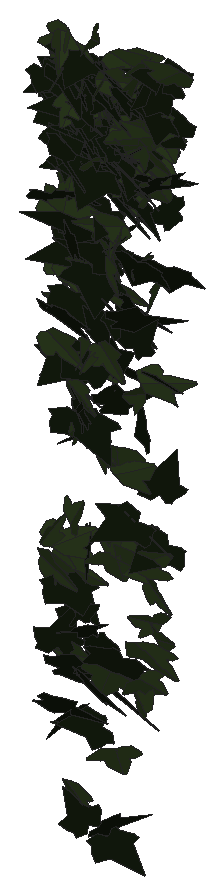
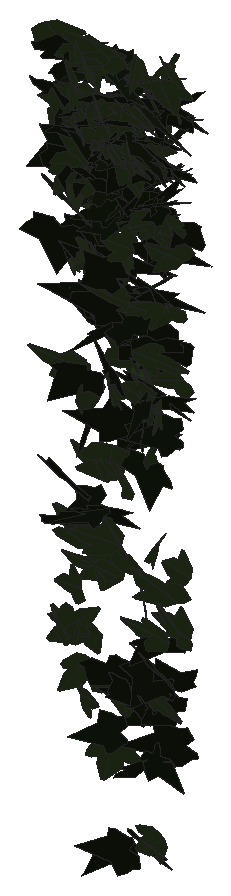
# SketchUp Ruby script. Lengths in millimetres.
U = 1.mm
M = Sketchup.active_model
def pt(a) = Geom::Point3d.new(a.map { |v| v * U })
def face(e, loops, mat)
  f = e.add_face(loops[0].map { |a| pt(a) })
  loops[1..].each { |l| e.add_face(l.map { |a| pt(a) }).erase! }
  f.material = f.back_material = mat if mat
  f
end
# faces: each face lists its corners as indices into pts; further lists are holes
def faces(e, pts, list, mat = nil) = list.each { |f| face(e, (f[0].is_a?(Array) ? f : [f]).map { |l| l.map { |i| pts[i] } }, mat) }
# xy, xz, yz: faces in a plane at the given z, y or x. An outline is a flat list of corners, or four numbers for a rectangle; further outlines are holes
def ring(l) = l.size == 4 ? [[l[0], l[1]], [l[2], l[1]], [l[2], l[3]], [l[0], l[3]]] : l.each_slice(2).to_a
def flat(e, list, mat, &to3) = list.each { |f| face(e, (f[0].is_a?(Array) ? f : [f]).map { |l| ring(l).map { |u, v| to3.(u, v) } }, mat) }
def xy(e, z, list, mat = nil) = flat(e, list, mat) { |x, y| [x, y, z] }
def xz(e, y, list, mat = nil) = flat(e, list, mat) { |x, z| [x, y, z] }
def yz(e, x, list, mat = nil) = flat(e, list, mat) { |y, z| [x, y, z] }
def lines(e, pts, list) = list.each { |a, b| e.add_line(pt(pts[a]), pt(pts[b])) }
# prism: a flat outline (further loops are holes) pulled along v
def prism(e, loops, v, mat = nil)
  f = face(e, loops, mat); d = Geom::Vector3d.new(v.map { |x| x * U })
  f.pushpull(f.normal.samedirection?(d) ? d.length : -d.length)
end
def box(e, o, s, mat = nil) = prism(e, [[o, [o[0] + s[0], o[1], o[2]], [o[0] + s[0], o[1] + s[1], o[2]], [o[0], o[1] + s[1], o[2]]]], [0, 0, s[2]], mat)
def at(x, y, z, deg = 0) = Geom::Transformation.translation(pt([x, y, z])) * Geom::Transformation.rotation(ORIGIN, Z_AXIS, deg.degrees)
def axes(o, x, y, z) = Geom::Transformation.new([*x, 0, *y, 0, *z, 0, *pt(o).to_a, 1])
def part(name) = M.definitions.add(name)
# library, detail: a bought-in or finely detailed component or shape, given as its bounding box
def library(name, o, s) = part(name).tap { |d| box(d.entities, o, s) }
def detail(e, o, s) = box(e.add_group.entities, o, s)
def put(e, d, t, mat = nil) = e.add_instance(d, t).tap { |i| i.material = mat if mat }
def group(e, t, mat = nil) = e.add_group.tap { |g| g.transformation = t; g.material = mat if mat }.entities
root = M.entities
M.materials.add("efeu1").color = [18, 25, 13]
M.materials.add("efeu2").color = [43, 57, 29]
c1 = part("ivyleaf_9")
p = [[39.1,54.8,31.7],[34.5,51.8,30.2],[-5.3,25.2,17.3],[-17.9,28.3,20.9],[-21.6,21.7,17],[-20.2,4.3,5.3],
  [-22.9,-0.3,2.5],[-17.1,-4,-0.6],[-2,-2.1,-1.2],[-0.7,-15.4,-10.1],[16.6,-22.3,-16.7],[21.1,-15.1,-12.5],
  [32.7,-10.7,-11],[46.1,-1.8,-6.6],[30.8,11.2,3.8]]
faces(c1.entities,p,[[0,1,2,3,4,5,6,7,8,9,10,11,12,13,14]],"efeu1")
c2 = part("ivyleaf_10")
p = [[0,12.8,-0.8],[-1.5,51.3,-10.9],[-4.9,51,-11.6],[-13.6,26.5,-7.3],[-13.2,15.9,-4.6],[-21.1,19.3,-7.2],
  [-29.5,16.3,-8.3],[-29.2,8.3,-6.2],[-19.7,-9.8,0.5],[-7.6,-13,4],[1,-12.2,5.8],[-0.4,51.1,-11.1],
  [-1.5,51.1,-10.9],[1,-12.4,5.9],[16.9,-12.4,3.5],[35.1,9.1,-5.1],[35,12.9,-6.1],[20.5,16.4,-4.9],
  [15.8,15,-3.8],[15.3,27.6,-7.1],[12.8,31.3,-7.8]]
faces(c2.entities,p,[[0,1,2,3,4,5,6,7,8,9,10],[11,12,0,13,14,15,16,17,18,19,20]],"efeu2")
put(root,c1,axes([2883.6,930,998.6],[-0.63134,-0.54805,-0.68858],[0.6758,0.58996,-0.64063],[1.53254,-0.48593,-0.00117]))
put(root,c1,axes([2814.2,927.9,1572.8],[0.42364,-0.6267,-0.48664],[-0.1479,0.48577,-0.66114],[1.50284,0.22447,0.07211]))
put(root,c1,axes([2824.3,923.5,489.8],[1.26667,0.04328,0.44833],[0.8493,0.04515,-0.66682],[-0.11628,0.80119,0.01336]))
put(root,c1,axes([2901.8,943.8,1419.4],[-1.00985,-0.67232,0.03547],[-0.0298,-0.03283,-0.85644],[1.281,-0.53078,0.00804]))
put(root,c2,axes([2826.4,921.6,772.8],[0.15116,-0.68397,0.61887],[-0.19573,0.61072,0.68816],[-1.74456,-0.12778,-0.02359]))
put(root,c1,axes([2953.8,925.9,1588.4],[1.11488,-0.41864,-0.46192],[-0.58225,0.35923,-0.71354],[1.03377,0.65382,0.09628]))
put(root,c2,axes([2840.4,927.7,1579.9],[0.4073,-0.77882,-0.38187],[-0.19853,0.36736,-0.80768],[1.63886,0.23806,-0.00294]))
put(root,c2,axes([2863.9,938.3,1531.9],[0.85208,0.61092,-0.37702],[-0.39134,-0.31658,-0.75716],[-1.30903,0.4923,-0.01905]))
put(root,c1,axes([2870.3,948.8,1520.5],[-0.85456,-0.2473,0.7023],[-1.02719,-0.45686,-0.50594],[0.97619,-0.69722,0.08242]))
put(root,c1,axes([2880.7,944,534.4],[0.58926,-0.49402,0.63243],[0.67074,-0.5253,-0.58287],[1.37218,0.46892,0.01333]))
put(root,c2,axes([2951.3,930.1,444.2],[-1.09314,-0.67103,-0.23331],[0.27125,0.18508,-0.88321],[1.32462,-0.59167,-0.01168]))
put(root,c1,axes([2871.9,924.2,1284.3],[0.04835,-0.26099,0.79603],[-0.14077,0.79259,0.26222],[-1.58814,-0.0782,0.00099]))
put(root,c2,axes([2990.5,933.8,779],[-1.40972,-0.27616,0.56116],[0.99911,0.19828,0.79051],[-0.64702,0.90787,-0.00196]))
put(root,c2,axes([2863.7,950.9,969.6],[-0.2876,0.2348,0.91607],[0.70199,-0.83959,0.27604],[1.65728,0.39638,0.04205]))
put(root,c2,axes([2860.2,943.9,1033.5],[-0.49701,0.25279,-0.71399],[0.86298,-0.55277,-0.36156],[-1.15467,-0.52194,0.03711]))
put(root,c1,axes([2974.1,948.1,840.1],[-1.35807,-0.37116,0.27644],[-0.45189,-0.14246,-0.80417],[0.75603,-0.75187,0.01591]))
put(root,c2,axes([2939.8,945.2,1332.4],[0.87647,-0.62325,0.36788],[0.40894,-0.29863,-0.77492],[1.31528,0.50817,-0.00421]))
put(root,c1,axes([2874.6,952.1,991.3],[0.04901,0.05203,0.86048],[-0.52356,-0.81536,0.05753],[1.55488,-0.27619,-0.00775]))
put(root,c2,axes([2916.1,948.1,1260.8],[-0.47084,0.36892,-0.73202],[0.59454,-0.6645,-0.44047],[-1.44239,-0.39433,0.0574]))
put(root,c2,axes([2990.2,943.2,1512.8],[-0.86521,-0.26856,0.6914],[-1.12787,-0.35615,-0.528],[0.84892,-0.7469,0.00316]))
put(root,c2,axes([2921.7,944.8,791.3],[0.75953,-0.51959,-0.47396],[0.58047,-0.36317,0.65495],[-1.20608,-0.502,0.01675]))
put(root,c1,axes([2896.5,927.4,303.6],[-1.21674,0.2044,-0.45949],[-0.82972,0.14522,0.67118],[0.47713,0.7738,-0.00459]))
put(root,c2,axes([2834.7,943.6,1628.3],[0.2442,0.75026,-0.38641],[-0.09263,-0.38362,-0.761],[-1.60347,0.13642,-0.01488]))
put(root,c1,axes([2873.3,931.5,1021.3],[1.00187,-0.39496,-0.54441],[-0.74918,0.37964,-0.65605],[1.03793,0.65526,0.05195]))
put(root,c2,axes([2849.6,935.9,1348.8],[1.69845,-0.0937,-0.04669],[0.08838,-0.00485,0.89732],[-0.17857,-0.89363,0.00002]))
put(root,c2,axes([2820.2,940.1,1106.6],[0.93583,-0.02456,0.68501],[1.30429,0.03446,-0.49069],[-0.02606,0.84252,0.04004]))
put(root,c1,axes([2829.5,932.6,1163.8],[1.59709,-0.04245,-0.15527],[-0.2952,0.00708,-0.84024],[0.08189,0.85338,-0.00075]))
put(root,c1,axes([2837.4,948.5,1442.3],[0.28172,-0.85599,0.04688],[0.01043,-0.04663,-0.86869],[1.63152,0.14811,-0.00254]))
put(root,c2,axes([2921.2,932.1,1593.4],[0.25219,-0.7053,-0.48967],[-0.0902,0.4887,-0.71674],[1.63163,0.13603,0.03606]))
put(root,c1,axes([2832.4,952.3,1561.9],[0.14112,-0.85093,0.24891],[0.16741,-0.24149,-0.85175],[1.67902,0.0956,0.06401]))
put(root,c2,axes([2867.8,946.3,1566],[0.84455,-0.69965,0.2326],[0.24622,-0.19337,-0.82849],[1.38145,0.4622,0.00547]))
put(root,c1,axes([2873.8,945.7,1317.7],[-0.68279,0.03215,-0.71065],[-0.88916,-0.61085,0.20822],[-1.02098,0.51048,0.29391]))
put(root,c1,axes([2987.2,935.7,1296.8],[1.16636,0.18657,-0.5871],[-1.06264,-0.18167,-0.64056],[-0.49536,0.82901,-0.00825]))
put(root,c2,axes([2910.5,946.9,1114.5],[0.97749,-0.20518,0.64934],[1.20621,-0.15352,-0.5498],[0.47415,0.81355,0.06002]))
put(root,c1,axes([2835.8,933.7,586.3],[-0.72,-0.35315,0.72211],[1.18478,0.3762,0.51011],[-0.96788,0.72321,0.08726]))
put(root,c1,axes([2934.8,935,287.1],[0.07191,-0.50189,-0.72315],[-0.11347,0.72069,-0.5033],[1.67144,0.07052,-0.00306]))
put(root,c2,axes([2931.1,940.1,564.4],[-1.62972,-0.1523,0.23958],[-0.44917,-0.04125,-0.86974],[0.3003,-0.88823,-0.00069]))
put(root,c2,axes([2937.6,944,1339.1],[0.55558,0.05176,-0.75248],[-1.43364,-0.02097,-0.29367],[-0.0729,0.80684,0.04064]))
put(root,c2,axes([2998,940.7,633.1],[-1.4185,0.07894,-0.51976],[0.97901,-0.07659,-0.74928],[-0.20649,-0.90542,0.01806]))
put(root,c1,axes([3025.2,955.6,815.4],[-1.22428,-0.5386,0.2061],[-0.30552,-0.12932,-0.83897],[1.05417,-0.66299,-0.00379]))
put(root,c1,axes([2841.3,937.3,547.7],[0.72496,-0.06687,0.7994],[1.5253,-0.00645,-0.38243],[0.06586,0.88549,0.05758]))
put(root,c1,axes([2828.2,931.8,1361.5],[1.45414,0.57437,-0.04188],[-0.06398,-0.02498,-0.95586],[-1.09417,0.76479,0.00023]))
put(root,c1,axes([2896.9,949.8,1238.1],[-1.19147,-0.38377,-0.42316],[0.66649,0.23817,-0.7341],[0.85899,-0.71712,-0.01735]))
put(root,c2,axes([3010.9,954.2,1259.6],[0.45099,-0.69809,0.4273],[0.31718,-0.39438,-0.73672],[1.52511,0.28845,0.02686]))
put(root,c1,axes([2957.9,932.5,1188.6],[0.73605,0.04129,0.82396],[1.48165,0.28292,-0.37958],[-0.51966,0.86513,0.08481]))
put(root,c1,axes([2848.9,950.2,1565.3],[-1.56216,0.04865,0.0752],[-0.14685,-0.03199,-0.82144],[-0.08656,-0.82362,0.03634]))
put(root,c1,axes([2977.7,940.3,1148.3],[-0.7019,0.59982,0.41627],[0.33559,-0.37938,0.70289],[1.34841,0.40664,0.04175]))
put(root,c1,axes([3002.3,961.5,1550.6],[-0.38626,-0.72127,0.44661],[0.19272,-0.47653,-0.72356],[1.60302,-0.1165,0.1946]))
put(root,c1,axes([2854.9,948.7,473.2],[-0.44054,0.56882,-0.55447],[0.41481,-0.50989,-0.61407],[-1.45378,-0.31785,-0.00719]))
put(root,c1,axes([2915.3,947,1599.6],[1.08297,-0.60883,-0.02337],[-0.01196,0.0261,-0.83324],[1.15952,0.56891,0.01323]))
put(root,c1,axes([2844.5,959,1071.5],[-1.07585,-0.54835,0.28499],[-0.3728,-0.20733,-0.78746],[1.1155,-0.59815,0.01169]))
put(root,c1,axes([2895.7,953.3,1555.3],[0.73341,-0.74928,0.17655],[0.17153,-0.15217,-0.84251],[1.45502,0.39562,0.01033]))
put(root,c1,axes([2942.1,949.2,593.5],[0.25796,0.30212,-0.80226],[-0.85908,-0.66536,-0.32683],[-1.38704,0.46829,0.05322]))
put(root,c1,axes([2965.3,944.1,850.6],[1.50653,-0.47803,-0.10684],[-0.16997,0.05879,-0.92471],[0.91661,0.79659,0.00413]))
put(root,c1,axes([2840.7,946.2,1552.8],[-0.68925,-0.3754,-0.68405],[0.89355,0.49752,-0.5216],[1.18615,-0.59293,-0.00456]))
put(root,c2,axes([2877,945,1107],[0.57076,-0.88965,-0.21557],[-0.12619,0.20514,-0.93883],[1.7376,0.30713,0.00263]))
put(root,c1,axes([2832.2,960.7,1442.8],[-0.31671,-0.83006,0.24522],[-0.08584,-0.24106,-0.84657],[1.64503,-0.17239,0.00304]))
put(root,c1,axes([2896.7,950.5,1086],[-1.69564,0.21213,0.14268],[-0.26476,0.03176,-0.91585],[-0.40822,-0.90174,0.00131]))
put(root,c2,axes([2939.6,944.5,769.8],[-1.2672,-0.61868,-0.19706],[0.27694,0.13289,-0.90889],[1.20432,-0.68154,0.00166]))
put(root,c1,axes([2856.5,962.5,1599.9],[-0.82221,-0.68704,0.20937],[0.02086,-0.25061,-0.79974],[1.36679,-0.40948,0.13815]))
put(root,c2,axes([2886.2,936.5,1082.6],[0.72199,-0.47502,0.61192],[-0.39414,0.59437,0.58977],[-1.42066,-0.4063,0.14736]))
put(root,c2,axes([2984.8,940.9,1494.5],[0.988,-0.39042,-0.56565],[-0.56333,0.51277,-0.62557],[1.18057,0.57142,0.17488]))
put(root,c2,axes([2890,957.6,1427],[0.09567,-0.79253,0.32776],[0.03504,-0.32725,-0.79412],[1.63187,0.05349,-0.00216]))
put(root,c1,axes([2932.9,950.6,1273.2],[-0.68948,0.10427,0.71846],[-1.31482,0.19728,-0.37698],[-0.42467,-0.78007,0.00069]))
put(root,c2,axes([2792,959.2,701.9],[0.01821,-0.11853,0.97857],[1.75075,-0.35055,-0.05146],[0.67408,0.91368,0.10721]))
put(root,c2,axes([2947.2,952.6,914.7],[1.11623,-0.21706,-0.6099],[1.10427,-0.18878,0.62514],[-0.54648,-0.82482,0.01743]))
put(root,c1,axes([3015.9,955.1,1590.7],[-1.453,0.21406,-0.26205],[0.49285,-0.04664,-0.79254],[-0.41451,-0.80582,-0.02374]))
put(root,c2,axes([2849.8,953.6,336.5],[-1.0113,0.47422,-0.42591],[0.57625,-0.30016,-0.71195],[-1.06751,-0.61128,0.01917]))
put(root,c2,axes([2861.4,933.3,813.5],[0.27901,0.03095,-0.92298],[0.11797,0.9321,0.0411],[1.75364,-0.06763,0.14408]))
put(root,c2,axes([2937.5,950.6,949.5],[-1.4976,-0.31021,-0.01961],[0.03485,0.00701,-0.84582],[0.59054,-0.7871,0.00019]))
put(root,c1,axes([2952.8,951.7,1327.2],[-0.73854,0.70584,-0.3151],[0.28637,-0.27685,-0.80548],[-1.443,-0.4162,0.00142]))
put(root,c2,axes([2928.2,938,1589.1],[0.17294,0.04144,0.86809],[0.65971,0.79867,-0.07441],[-1.51678,0.3521,0.06661]))
put(root,c1,axes([2809.1,953.1,1521.1],[0.74569,-0.69102,-0.30617],[-0.23141,0.28275,-0.79375],[1.41972,0.40904,0.03143]))
put(root,c1,axes([2907.9,969.2,1344],[-0.43275,-0.66168,0.42526],[-0.26954,-0.40099,-0.69966],[1.47251,-0.26786,-0.0031]))
put(root,c1,axes([2939.4,964.9,1426.1],[0.56434,-0.64631,0.47825],[0.45894,-0.41478,-0.71005],[1.45975,0.38027,0.03835]))
put(root,c2,axes([2826.1,955.5,1629.5],[1.00689,-0.65103,-0.10714],[-0.11877,0.08734,-0.83886],[1.25007,0.53268,0.0066]))
put(root,c2,axes([2864.9,947.5,571.8],[0.55778,-0.1675,-0.75225],[-1.13832,0.45809,-0.33503],[0.92496,0.66477,0.04132]))
put(root,c2,axes([2903.9,956.7,1288.9],[-0.80575,0.58806,-0.38068],[0.4475,-0.29971,-0.72447],[-1.25589,-0.48408,-0.01391]))
put(root,c1,axes([2855.2,944.9,1558.9],[0.65688,0.03695,-0.78352],[-1.44849,0.2229,-0.32475],[0.36122,0.82664,0.12259]))
put(root,c2,axes([2989.9,945,575.4],[-0.76231,-0.55747,-0.63228],[0.64586,0.53415,-0.68593],[1.46853,-0.5243,-0.02654]))
put(root,c2,axes([2810,968,714.5],[0.02654,-0.19207,-0.81099],[0.7861,-0.70289,0.17357],[-1.37767,-0.40477,0.08342]))
put(root,c1,axes([2887.3,971,448.4],[-0.05862,-0.60233,-0.52802],[-0.05029,-0.52736,0.60312],[-1.52364,0.04058,0.00041]))
put(root,c1,axes([2949.3,972.6,1430.4],[-0.31138,-0.68831,0.45102],[-0.0531,-0.45495,-0.70442],[1.56528,-0.15236,0.06582]))
put(root,c2,axes([2944.6,945.5,797],[-0.17975,-0.48182,0.82601],[0.41668,0.79709,0.48998],[-1.77163,0.23636,0.03143]))
put(root,c1,axes([2848.7,972.1,1396.3],[-0.21288,0.03204,0.78495],[-0.03033,-0.7928,0.03009],[1.49485,-0.01152,0.11239]))
put(root,c2,axes([2989.5,950.5,526.5],[0.64213,-0.2002,0.78548],[-1.24174,0.43781,0.39184],[-0.91547,-0.73427,0.01947]))
put(root,c2,axes([2824.4,955,751.5],[1.25075,0.14401,-0.65962],[1.22971,0.13287,0.67275],[0.37274,-0.92159,-0.00608]))
put(root,c2,axes([2965.2,962.8,1594.8],[0.0757,-0.84546,-0.01075],[0.02372,0.01134,-0.8463],[1.60904,0.03961,0.01298]))
put(root,c2,axes([2909.6,962.7,1220.7],[0.02159,-0.05015,0.84447],[1.60904,0.03013,-0.00957],[-0.05615,0.84401,0.05051]))
put(root,c2,axes([2886.5,974.3,921.3],[0.05333,-0.16305,-0.82191],[0.72773,-0.72927,0.15771],[-1.41903,-0.38012,0.04999]))
put(root,c1,axes([2920,965,1202.2],[1.09353,-0.35446,0.51902],[0.80851,-0.29923,-0.67465],[0.88156,0.71413,-0.02507]))
put(root,c2,axes([2896.4,963.2,1529],[-1.34299,-0.39815,0.0833],[-0.02792,-0.14177,-0.80193],[0.77367,-0.69626,0.11566]))
put(root,c1,axes([2922.2,964.9,1475],[-1.14841,0.11226,0.59349],[-1.1157,0.09324,-0.61366],[-0.27692,-0.84121,0.01119]))
put(root,c1,axes([3026.4,955.4,1293.1],[1.2457,0.36972,-0.41326],[-0.66752,-0.21914,-0.75156],[-0.8174,0.74241,-0.01604]))
put(root,c1,axes([2868.5,966,1159.1],[-0.7847,-0.12852,-0.71929],[1.31629,0.19778,-0.43178],[0.44859,-0.80514,0.00875]))
put(root,c2,axes([2975.2,964.6,1619.4],[-0.14883,-0.85343,0.02497],[0.04423,-0.0272,-0.85662],[1.62434,-0.07745,0.02561]))
put(root,c1,axes([2911.2,945.2,295.3],[0.10617,0.62679,-0.58324],[-0.08814,0.58583,0.62515],[1.62708,-0.00917,0.07192]))
put(root,c2,axes([2890.1,965.6,1079.4],[1.14695,0.19496,-0.51579],[-0.96821,-0.09817,-0.6315],[-0.40484,0.78713,0.04899]))
put(root,c1,axes([2837.4,973.9,1489.5],[0.35597,-0.76002,0.2687],[0.07465,-0.26693,-0.78232],[1.53239,0.18956,-0.02431]))
put(root,c2,axes([2838.3,956.9,1229.6],[0.84529,0.17752,0.63939],[1.01954,0.35813,-0.47155],[-0.74531,0.69124,0.08011]))
put(root,c2,axes([3032.6,966.7,1625.8],[-1.07519,-0.36197,0.49649],[-0.79648,-0.26714,-0.67095],[0.85619,-0.70306,-0.00068]))
put(root,c1,axes([2951.3,971.8,1384.7],[0.50801,-0.78194,0.14398],[0.10283,-0.13369,-0.82621],[1.50972,0.27222,0.00783]))
put(root,c2,axes([2979.7,958.6,1522.9],[1.202,-0.41535,-0.36935],[-0.35252,0.36983,-0.73262],[0.99737,0.63128,0.18618]))
put(root,c2,axes([2813.4,949.3,1315.1],[0.63683,0.38881,-0.75083],[0.96049,0.55604,0.51284],[1.29113,-0.60542,-0.01118]))
put(root,c1,axes([2999,978.5,1591.5],[0.05111,-0.08138,-0.82508],[0.52345,-0.77789,0.08568],[-1.48856,-0.27634,0.0018]))
put(root,c1,axes([2855.7,974,1252.5],[-1.31586,-0.18242,0.44208],[-0.7973,-0.14383,-0.71453],[0.43902,-0.80794,0.02739]))
put(root,c1,axes([2842.3,964,1404.8],[-0.68233,-0.71787,0.36931],[0.43002,0.29872,0.79999],[-1.47505,0.41916,0.06238]))
put(root,c2,axes([2966.3,976.1,1513],[-0.47461,-0.52013,0.57878],[-0.07519,-0.59853,-0.55489],[1.47907,-0.19733,0.15751]))
put(root,c1,axes([2912.2,970.8,1080.1],[-0.11962,0.3839,0.76711],[0.2337,-0.75722,0.38901],[1.61577,0.13794,0.00052]))
put(root,c1,axes([2829.2,961.9,680],[-0.07901,-0.64728,-0.63371],[0.11657,0.63092,-0.64845],[1.72008,-0.07249,0.01483]))
put(root,c2,axes([2990.8,977.9,658.4],[-0.50052,-0.24108,-0.73681],[-0.79922,-0.60973,0.34938],[-1.24026,0.4902,0.07221]))
put(root,c2,axes([2939.3,958.8,754],[0.81086,-0.04888,-0.73488],[1.38378,0.16328,0.41067],[0.2235,-0.83361,0.12353]))
put(root,c1,axes([2911.9,959.2,1544.6],[-0.95411,0.59775,0.24254],[-0.41055,0.13415,-0.77648],[-1.15704,-0.54051,0.07551]))
put(root,c2,axes([2826.3,962.1,1230.6],[1.20565,0.48756,0.24177],[0.36485,0.14733,-0.79939],[-0.96936,0.66186,-0.00016]))
put(root,c1,axes([2911.5,964.2,1461.7],[1.32281,-0.40928,0.03289],[0.05974,-0.01152,-0.80658],[0.77917,0.69573,0.006]))
put(root,c2,axes([2912.8,975.1,1473.2],[0.41571,-0.67264,0.43846],[0.28445,-0.41239,-0.70711],[1.50143,0.26437,0.01256]))
put(root,c2,axes([2998.7,972.4,633.8],[-0.82647,0.20169,0.66637],[1.10029,-0.33315,0.47759],[0.73833,0.72224,0.0342]))
put(root,c1,axes([2873.4,978.9,1185.1],[1.32483,-0.36773,-0.47611],[0.79691,-0.22665,0.78726],[-0.82208,-0.81233,-0.00412]))
put(root,c2,axes([2979.7,973.6,720.5],[0.35503,-0.26248,0.75231],[1.34848,-0.2988,-0.27994],[0.69368,0.71518,0.15914]))
put(root,c1,axes([2864.3,951.8,953.1],[0.26408,0.83297,0.17081],[0.05441,0.1684,-0.84445],[-1.61738,0.14167,-0.00052]))
put(root,c1,axes([2926.6,965.8,1470.2],[1.26502,-0.45827,0.05261],[0.10344,-0.01384,-0.80712],[0.8718,0.66661,0.01942]))
put(root,c2,axes([2828.3,965,1605.6],[1.55655,0.08517,-0.1711],[-0.34766,0.12717,-0.80986],[-0.10699,0.82583,0.14236]))
put(root,c2,axes([3014.8,977.1,1530.8],[-0.2002,-0.61205,0.52001],[0.11064,-0.52888,-0.61073],[1.52451,-0.04199,0.11261]))
put(root,c2,axes([2897.2,961,1541],[-0.65696,0.73963,0.09539],[-0.08959,0.08329,-0.81618],[-1.41649,-0.3483,0.00738]))
put(root,c2,axes([2913.9,965.7,1547.7],[-1.2415,-0.50228,-0.01359],[0.05667,-0.0164,-0.8227],[0.95461,-0.65226,0.03116]))
put(root,c1,axes([3004.9,947.8,1432.5],[0.90821,0.52153,0.62438],[0.78537,0.46866,-0.70685],[-1.33435,0.63082,0.00894]))
put(root,c2,axes([3016,957,1456.9],[0.1227,0.00912,-0.85901],[-1.21317,0.57799,-0.0417],[1.09605,0.63873,0.05001]))
put(root,c1,axes([2850.9,952,608.8],[0.80211,0.65574,0.26194],[0.27504,0.21849,-0.77949],[-1.31544,0.44553,-0.00326]))
put(root,c2,axes([2971.7,966.7,1513.7],[-1.13275,-0.54617,0.01409],[-0.01916,-0.00987,-0.8078],[1.03965,-0.59527,0.00046]))
put(root,c2,axes([2998.1,963.2,1510.2],[1.23505,0.30322,0.3824],[0.57523,0.24981,-0.711],[-0.72923,0.71059,0.08678]))
put(root,c1,axes([2960.5,976.3,1521.9],[-0.47627,-0.75614,-0.11815],[0.1158,0.10426,-0.79609],[1.45195,-0.25635,0.02473]))
put(root,c1,axes([3029.5,978.1,1599.2],[-0.44658,-0.01298,0.79596],[-1.41259,-0.29644,-0.22364],[0.54775,-0.77507,0.0722]))
put(root,c1,axes([2910.6,967.5,1587.4],[-1.14382,0.58208,-0.13311],[0.07689,-0.14879,-0.83305],[-1.1338,-0.59731,0.07779]))
put(root,c1,axes([2841,983.5,1379.9],[-0.6734,-0.60007,0.3717],[0.04298,-0.42519,-0.66494],[1.34271,-0.28734,0.2077]))
put(root,c1,axes([2855,980.9,766],[-0.5041,0.10889,-0.94777],[1.55952,-0.47774,-0.28389],[-0.92979,-0.86034,0.03769]))
put(root,c1,axes([2838,969.9,1177.9],[-0.38053,-0.65934,-0.48241],[0.26703,0.46155,-0.68899],[1.53176,-0.24426,0.00027]))
put(root,c1,axes([2862.9,982.3,1455.8],[-0.03768,-0.7303,0.3051],[-0.01722,-0.30496,-0.73057],[1.50622,-0.02175,-0.00072]))
put(root,c1,axes([2844.1,984.3,1406.2],[-0.98147,-0.29361,0.53354],[-0.58554,-0.47775,-0.56028],[1.00025,-0.56777,0.19554]))
put(root,c1,axes([2817.2,976.8,1476.6],[-0.77173,-0.56768,-0.40989],[0.78693,0.18812,-0.66958],[1.07544,-0.54502,0.19582]))
put(root,c2,axes([2991.2,965.1,1079.7],[0.62668,0.01072,-0.79971],[1.50941,0.10729,0.32799],[0.19654,-0.85817,0.03102]))
put(root,c1,axes([2804.3,971.5,1033.4],[1.31953,-0.47552,0.18356],[0.29328,-0.09985,-0.84071],[0.9247,0.71022,0.0047]))
put(root,c1,axes([2918.1,975.8,1556.1],[-0.70938,-0.6506,-0.34101],[0.31828,0.2972,-0.74981],[1.3613,-0.40852,-0.0024]))
put(root,c2,axes([2901.6,957.4,1306.7],[0.04474,-0.56616,0.73719],[-0.1011,0.7354,0.56648],[-1.76615,-0.05644,-0.01376]))
put(root,c2,axes([2864.2,975.1,1515.6],[1.2764,-0.44343,0.1329],[0.19876,-0.08299,-0.80392],[0.8583,0.67865,-0.01147]))
put(root,c1,axes([2993.5,961.7,1492.3],[-0.0377,0.81068,-0.01872],[0.00069,-0.01872,-0.81093],[-1.5433,-0.01981,0.0001]))
put(root,c2,axes([2930.2,963.8,1616.5],[0.87623,0.15133,0.70044],[1.06149,0.44707,-0.46319],[-0.85633,0.70902,0.14256]))
put(root,c2,axes([2948.8,969.7,1401.9],[1.02321,0.61433,0.05948],[0.06475,0.04926,-0.81634],[-1.17288,0.53866,0.00682]))
put(root,c1,axes([2847.4,978.8,1477.3],[0.09664,-0.79132,-0.07383],[0.21198,0.08034,-0.78445],[1.49766,0.03969,0.1158]))
put(root,c2,axes([2955.8,987.9,1037],[-0.11757,-0.25957,-0.81976],[-0.42619,-0.78866,0.26659],[-1.58004,0.23204,-0.01091]))
put(root,c1,axes([2854.3,980.6,1513.9],[-1.2243,-0.47837,-0.1466],[0.22706,0.08524,-0.80165],[0.92476,-0.65425,0.00275]))
put(root,c1,axes([2851.9,975.7,1495],[-1.48065,0.21074,-0.10051],[0.19408,-0.00785,-0.80579],[-0.39974,-0.78441,-0.01894]))
put(root,c2,axes([2982.4,972.7,1505.7],[0.30972,-0.81461,-0.12345],[-0.03466,0.12224,-0.83068],[1.56768,0.16364,0.00603]))
put(root,c1,axes([2855.7,958.4,630.8],[-1.16337,0.51618,-0.29726],[-0.43371,0.19088,0.80006],[1.04741,0.65237,0.00111]))
put(root,c1,axes([2860.1,978,1272],[-1.50939,0.12274,-0.25248],[0.47509,-0.03786,-0.80252],[-0.24445,-0.83144,-0.00072]))
put(root,c2,axes([2955.8,975.6,1543.9],[1.60748,-0.27428,-0.06915],[-0.12014,0.02949,-0.888],[0.52477,0.84693,0.00853]))
put(root,c1,axes([2902.7,977.7,1465.2],[0.81975,-0.65108,0.16732],[0.4726,-0.03056,-0.75817],[1.18891,0.46107,0.18601]))
put(root,c1,axes([2832.2,970.8,1407.2],[1.38046,-0.30458,-0.06604],[-0.10641,0.03739,-0.78659],[0.58353,0.72738,0.01279]))
put(root,c1,axes([2912.8,975.5,1376.4],[1.17712,-0.54837,-0.00221],[-0.00321,0.00142,-0.82659],[1.04367,0.6185,-0.00006]))
put(root,c1,axes([2955.7,992.7,975.3],[-0.06848,-0.16594,0.94635],[-0.41306,-0.92113,-0.16976],[1.78131,-0.21998,-0.00299]))
put(root,c2,axes([2948.2,974.3,1501.8],[1.22339,0.51287,0.03106],[0.05139,0.01595,-0.82232],[-0.97652,0.64336,-0.00437]))
put(root,c1,axes([2910.8,984.8,1536.9],[0.28219,-0.78854,0.15368],[0.05326,-0.15111,-0.80236],[1.52806,0.15089,-0.00041]))
put(root,c1,axes([2931.5,968.6,1454.7],[-0.75978,-0.5584,0.61929],[0.67946,0.50604,0.68642],[-1.4342,0.53556,-0.00288]))
put(root,c2,axes([2909.8,982.5,1081.1],[0.84597,-0.60257,0.35047],[0.48398,-0.24684,-0.74693],[1.23525,0.50939,0.05263]))
put(root,c2,axes([2934.1,977.9,1503.5],[-1.10601,-0.36356,0.42331],[-0.70439,-0.20626,-0.68524],[0.79476,-0.68874,-0.01823]))
put(root,c2,axes([2969.7,958.9,1270.5],[0.34048,-0.03798,0.82931],[-0.45167,0.8106,0.08832],[-1.51405,-0.25036,0.16015]))
put(root,c2,axes([2889.7,977.8,1457.3],[1.50955,-0.07394,-0.01763],[-0.03393,-0.00127,-0.7966],[0.14063,0.79336,-0.00292]))
put(root,c1,axes([2870.8,987.2,1506],[-0.98811,-0.62151,-0.03766],[0.22407,-0.04984,-0.80056],[1.16365,-0.51816,0.12218]))
put(root,c1,axes([2923,969,1171.1],[0.50361,-0.49015,-0.62261],[-0.21497,0.62638,-0.54111],[1.49269,0.25557,0.13213]))
put(root,c1,axes([2875.7,981.4,586.8],[-0.45891,-0.05773,-0.76486],[1.45551,0.04346,-0.24438],[0.11207,-0.80079,0.04187]))
put(root,c1,axes([2911.7,991.2,1401],[-0.18356,-0.52638,0.59874],[0.21443,-0.60605,-0.51465],[1.50204,0.02219,0.14664]))
put(root,c1,axes([3040.2,970.5,1521],[-0.73436,0.27044,0.67565],[-0.99436,0.42944,-0.47026],[-0.96423,-0.64883,-0.02962]))
put(root,c2,axes([2954.1,973,1622.4],[0.9437,0.16725,0.65925],[1.16793,0.24174,-0.5229],[-0.5581,0.78869,0.02047]))
put(root,c2,axes([2993.5,977.9,1585.7],[0.80405,-0.7153,-0.04041],[0.08147,0.07203,-0.82749],[1.36109,0.41824,0.0734]))
put(root,c1,axes([2978.1,986.9,1490.8],[-0.89193,-0.66084,-0.06581],[0.1476,0.02553,-0.80871],[1.25529,-0.47256,0.04833]))
put(root,c2,axes([2854.8,979.5,1499.7],[-1.17646,-0.37302,0.40934],[-0.65507,-0.22182,-0.7219],[0.82572,-0.70743,0.01051]))
put(root,c2,axes([2854.4,974.7,1153.1],[0.11347,-0.02944,-0.83382],[-1.52979,0.22209,-0.06531],[0.42573,0.80591,-0.01246]))
put(root,c1,axes([2898,969.5,1436.9],[0.9773,0.45053,-0.41731],[-0.74331,-0.1802,-0.67513],[-0.90195,0.63668,0.10421]))
put(root,c1,axes([2970,969.3,1082.9],[1.62018,0.12056,-0.12346],[-0.23312,-0.01554,-0.85979],[-0.23132,0.86006,0.00177]))
put(root,c2,axes([2935.7,979.3,1482.3],[1.4762,-0.25844,-0.09532],[-0.17233,0.02979,-0.81756],[0.49512,0.78091,-0.00036]))
put(root,c2,axes([2840.7,979,1386.4],[-1.19796,-0.37013,0.31975],[-0.52951,-0.15765,-0.73019],[0.76562,-0.68817,-0.0047]))
put(root,c1,axes([2883.5,993.4,1393.6],[0.61309,-0.46197,-0.56698],[0.5797,-0.47851,0.56294],[-1.26545,-0.44302,-0.01681]))
put(root,c2,axes([2824,982.1,695.4],[0.00538,0.00453,-0.79912],[1.35293,-0.36508,0.00044],[-0.69481,-0.71085,-0.00532]))
put(root,c2,axes([2973.4,990.3,1396.4],[0.22742,-0.7861,0.55869],[0.23908,-0.54548,-0.79438],[1.81982,0.1699,0.03454]))
put(root,c2,axes([2973.1,978.8,1549.2],[-0.22584,-0.8194,-0.02635],[0.0294,0.02439,-0.82787],[1.56002,-0.11908,0.01179]))
put(root,c2,axes([2898.3,975.4,1542],[-1.33128,-0.4216,-0.0796],[0.11287,0.05578,-0.81655],[0.80874,-0.7018,-0.01708]))
put(root,c2,axes([2838,975.2,1388.1],[-1.37577,0.30848,-0.06623],[0.10832,-0.03537,-0.78587],[-0.59063,-0.72504,0.01016]))
put(root,c1,axes([2906.2,963.7,1013.8],[0.31449,0.12876,0.87724],[1.47008,0.41719,-0.20673],[-0.82844,0.78918,-0.03384]))
put(root,c2,axes([2933.2,984.9,1537],[-0.30121,-0.75081,0.27557],[-0.03782,-0.27714,-0.76649],[1.52169,-0.15551,0.0355]))
put(root,c1,axes([2861.8,985.5,1490.1],[-1.29581,0.24372,-0.34248],[0.46026,-0.30612,-0.69862],[-0.65436,-0.69796,0.18682]))
put(root,c1,axes([2908.6,979,1265.3],[1.18873,0.15303,-0.47673],[0.83675,0.19707,0.63928],[0.45596,-0.76063,0.06972]))
put(root,c1,axes([2991.4,970.1,1429.3],[0.80569,0.69725,-0.21629],[-0.20803,-0.18667,-0.81569],[-1.37372,0.4372,-0.00333]))
put(root,c2,axes([2924.3,990.3,1491.8],[-0.39144,0.32932,-0.7003],[0.35314,-0.68249,-0.37544],[-1.42986,-0.25871,0.09899]))
put(root,c2,axes([2934.3,981.9,1546.4],[0.40705,-0.79503,0.01086],[0.02083,-0.0083,-0.82325],[1.51309,0.21399,0.00841]))
put(root,c2,axes([2835.6,965,1063.7],[0.189,-0.29894,-0.80701],[-0.08666,0.8094,-0.30543],[1.6356,0.07743,0.07707]))
put(root,c1,axes([2848.9,976.7,1559.6],[-1.0549,0.61063,0.06662],[-0.17821,0.00469,-0.82204],[-1.15539,-0.55825,0.06596]))
put(root,c1,axes([2918.4,989.3,1522.4],[-0.92211,-0.62371,-0.1688],[0.26489,0.10529,-0.78854],[1.20087,-0.50215,0.04433]))
put(root,c2,axes([2914.3,978.9,1505.9],[-0.65908,-0.70029,-0.17635],[0.19182,0.1468,-0.78085],[1.36095,-0.35982,0.02465]))
put(root,c1,axes([3026,978.8,1380.1],[-1.13619,0.5547,0.02639],[-0.04014,0.01607,-0.81491],[-1.05613,-0.59736,0.00258]))
put(root,c1,axes([2895.3,985.8,1505.3],[0.497,-0.7518,-0.13057],[-0.10279,0.11945,-0.79578],[1.44861,0.26641,-0.01167]))
put(root,c1,axes([2898.2,982.7,511.2],[1.29885,-0.45545,0.16105],[0.25874,-0.08641,-0.82047],[0.88225,0.69586,0.00352]))
put(root,c2,axes([2989.3,975.6,1416.7],[-0.79609,-0.63523,-0.40609],[0.49487,0.31436,-0.75958],[1.34686,-0.49097,0.03906]))
put(root,c2,axes([2876.4,986,1459.1],[-0.35824,-0.77605,0.16166],[-0.07011,-0.15741,-0.79855],[1.50706,-0.1918,0.00128]))
put(root,c2,axes([2916.2,982.1,1472.8],[1.0542,-0.56546,-0.20766],[-0.2695,0.15197,-0.79154],[1.11433,0.5717,0.00502]))
put(root,c2,axes([2977.1,987.8,1449.9],[0.88055,0.52111,-0.41546],[-0.5376,-0.30476,-0.69682],[-1.14884,0.54203,0.00764]))
put(root,c1,axes([2878.6,971.3,1464.5],[1.17119,0.5123,0.01662],[0.02361,0.01108,-0.80071],[-0.97523,0.6155,0.00058]))
put(root,c2,axes([2870.4,971.1,1627.8],[-0.08263,-0.54945,-0.64357],[0.07749,0.64232,-0.55113],[1.60866,-0.05916,-0.00651]))
put(root,c1,axes([2901.9,985.9,1360.4],[0.97691,-0.61052,0.01301],[0.00597,-0.01437,-0.7976],[1.16219,0.51326,-0.00685]))
put(root,c1,axes([2851.5,976.3,1074],[0.97049,-0.33187,-0.57273],[-0.93129,0.29789,-0.60828],[0.84841,0.70662,-0.01256]))
put(root,c1,axes([2933.4,989.9,1424.4],[-1.13749,-0.19423,-0.50469],[0.96837,0.0528,-0.62288],[0.34859,-0.78047,0.08346]))
put(root,c1,axes([3002,972.4,891.1],[-1.2379,0.63245,0.13165],[0.15933,-0.10272,0.9071],[1.21912,0.65562,0.01512]))
put(root,c1,axes([2818.2,989.9,1286.7],[0.2806,-0.7677,-0.05262],[0.01518,0.0551,-0.78152],[1.46443,0.14653,0.01818]))
put(root,c2,axes([2862.9,984.4,1505.3],[-0.11917,-0.81239,-0.06941],[-0.04721,0.07148,-0.81424],[1.55106,-0.06024,-0.03012]))
put(root,c1,axes([2860.1,978.3,1509.3],[-0.49638,0.76593,-0.10414],[0.08645,-0.09454,-0.80902],[-1.46859,-0.26444,-0.01242]))
